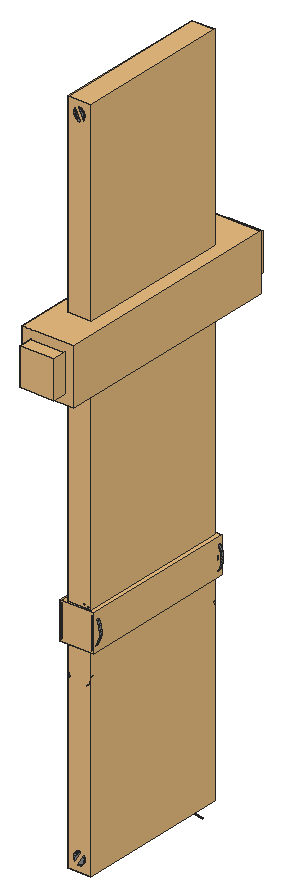
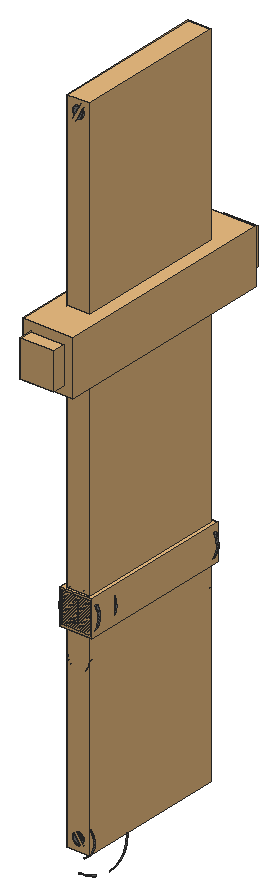
# SketchUp Ruby script. Lengths in inches.
U = 1.inch
M = Sketchup.active_model
def pt(a) = Geom::Point3d.new(a.map { |v| v * U })
def face(e, loops, mat)
  f = e.add_face(loops[0].map { |a| pt(a) })
  loops[1..].each { |l| e.add_face(l.map { |a| pt(a) }).erase! }
  f.material = f.back_material = mat if mat
  f
end
# faces: each face lists its corners as indices into pts; further lists are holes
def faces(e, pts, list, mat = nil) = list.each { |f| face(e, (f[0].is_a?(Array) ? f : [f]).map { |l| l.map { |i| pts[i] } }, mat) }
# xy, xz, yz: faces in a plane at the given z, y or x. An outline is a flat list of corners, or four numbers for a rectangle; further outlines are holes
def ring(l) = l.size == 4 ? [[l[0], l[1]], [l[2], l[1]], [l[2], l[3]], [l[0], l[3]]] : l.each_slice(2).to_a
def flat(e, list, mat, &to3) = list.each { |f| face(e, (f[0].is_a?(Array) ? f : [f]).map { |l| ring(l).map { |u, v| to3.(u, v) } }, mat) }
def xy(e, z, list, mat = nil) = flat(e, list, mat) { |x, y| [x, y, z] }
def xz(e, y, list, mat = nil) = flat(e, list, mat) { |x, z| [x, y, z] }
def yz(e, x, list, mat = nil) = flat(e, list, mat) { |y, z| [x, y, z] }
def lines(e, pts, list) = list.each { |a, b| e.add_line(pt(pts[a]), pt(pts[b])) }
# prism: a flat outline (further loops are holes) pulled along v
def prism(e, loops, v, mat = nil)
  f = face(e, loops, mat); d = Geom::Vector3d.new(v.map { |x| x * U })
  f.pushpull(f.normal.samedirection?(d) ? d.length : -d.length)
end
def box(e, o, s, mat = nil) = prism(e, [[o, [o[0] + s[0], o[1], o[2]], [o[0] + s[0], o[1] + s[1], o[2]], [o[0], o[1] + s[1], o[2]]]], [0, 0, s[2]], mat)
def at(x, y, z, deg = 0) = Geom::Transformation.translation(pt([x, y, z])) * Geom::Transformation.rotation(ORIGIN, Z_AXIS, deg.degrees)
def axes(o, x, y, z) = Geom::Transformation.new([*x, 0, *y, 0, *z, 0, *pt(o).to_a, 1])
def part(name) = M.definitions.add(name)
# library, detail: a bought-in or finely detailed component or shape, given as its bounding box
def library(name, o, s) = part(name).tap { |d| box(d.entities, o, s) }
def detail(e, o, s) = box(e.add_group.entities, o, s)
def put(e, d, t, mat = nil) = e.add_instance(d, t).tap { |i| i.material = mat if mat }
def group(e, t, mat = nil) = e.add_group.tap { |g| g.transformation = t; g.material = mat if mat }.entities
root = M.entities
M.materials.add("Material \#1").color = [140, 140, 140]
c1 = library("3DGeom~4_Defintion",[-18.02,-499.97,-221.16],[36.04,1000,262.12])
c2 = part("3DGeom~5_Defintion")
xy(c2.entities,-225.24,[[-0.79,-499.98,-2.33,-499.64,7.45,-496.14],[-0.79,-499.98,7.45,-496.14,1.58,-499.88],[1.58,-499.88,7.45,-496.14,3.84,-499.16],[-2.33,-499.64,7.4,-485.75,7.45,-496.14],[3.84,-499.16,7.45,-496.14,5.85,-497.89],
  [7.45,-496.14,7.4,-485.75,8.24,-487.08],[7.45,-496.14,8.24,-487.08,8.96,-489.34],[7.45,-496.14,8.96,-489.34,9.0625,-491.71],[7.45,-496.14,9.0625,-491.71,8.55,-494.03],[-7.4,-496.08,-8.24,-494.76,2.32,-482.2],
  [-8.24,-494.76,-8.96,-492.5,2.32,-482.2],[-8.96,-492.5,-9.0625,-490.125,2.32,-482.2],[-9.0625,-490.125,-8.55,-487.81,2.32,-482.2],[-8.55,-487.81,-7.45,-485.7,2.32,-482.2],[-7.45,-485.7,-5.85,-483.95,2.32,-482.2],
  [-5.85,-483.95,-3.84,-482.68,2.32,-482.2],[-3.84,-482.68,-1.58,-481.96,2.32,-482.2],[2.32,-482.2,-1.58,-481.96,0.79,-481.86],[0,481.82,-2.35,482.13,-6.92,496.71],[0,481.82,-6.92,496.71,1.55,482.04],
  [-2.35,482.13,-4.55,483.04,-6.92,496.71],[-4.55,483.04,-6.43,484.49,-6.92,496.71],[-6.43,484.49,-7.88,486.37,-6.92,496.71],[6.92,485.12,-1.55,499.8125,7.88,495.47],[6.92,485.12,7.88,495.47,7.88,486.37],
  [-7.88,486.37,-8.79,488.57,-6.92,496.71],[7.88,486.37,7.88,495.47,8.79,488.57],[-8.79,488.57,-9.1,490.92,-6.92,496.71],[8.79,488.57,7.88,495.47,9.1,490.92],[-9.1,490.92,-8.79,493.28,-6.92,496.71],
  [9.1,490.92,7.88,495.47,8.79,493.28],[-8.79,493.28,-7.88,495.47,-6.92,496.71],[7.88,495.47,-1.55,499.8125,0,500.02],[7.88,495.47,0,500.02,2.35,499.71],[7.88,495.47,2.35,499.71,4.55,498.8],
  [7.88,495.47,4.55,498.8,6.43,497.35]],"Material \#1")
xy(c2.entities,-221.57,[[-2.33,-499.64,-5.22,-498.37,7.4,-485.75],[-5.22,-498.37,-7.4,-496.08,5.22,-483.47],[-5.22,-498.37,5.22,-483.47,7.4,-485.75],[-7.4,-496.08,2.32,-482.2,5.22,-483.47],[1.55,482.04,-6.92,496.71,-4.55,498.8],
  [1.55,482.04,-4.55,498.8,4.55,483.04],[4.55,483.04,-4.55,498.8,-1.55,499.8125],[4.55,483.04,-1.55,499.8125,6.92,485.12]],"Material \#1")
xy(c2.entities,38.05,[[-2.33,-499.64,7.4,-485.75,-5.22,-498.37],[-5.22,-498.37,5.22,-483.47,-7.4,-496.08],[-5.22,-498.37,7.4,-485.75,5.22,-483.47],[-7.4,-496.08,5.22,-483.47,2.32,-482.2],[1.55,482.04,-4.55,498.8,-6.92,496.71],
  [1.55,482.04,4.55,483.04,-4.55,498.8],[4.55,483.04,-1.55,499.8125,-4.55,498.8],[4.55,483.04,6.92,485.12,-1.55,499.8125]],"Material \#1")
xy(c2.entities,41.72,[[-0.79,-499.98,7.45,-496.14,-2.33,-499.64],[-0.79,-499.98,1.58,-499.88,7.45,-496.14],[1.58,-499.88,3.84,-499.16,7.45,-496.14],[-2.33,-499.64,7.45,-496.14,7.4,-485.75],[3.84,-499.16,5.85,-497.89,7.45,-496.14],
  [7.45,-496.14,8.24,-487.08,7.4,-485.75],[7.45,-496.14,8.55,-494.03,9.0625,-491.71],[7.45,-496.14,8.96,-489.34,8.24,-487.08],[7.45,-496.14,9.0625,-491.71,8.96,-489.34],[-7.4,-496.08,2.32,-482.2,-8.24,-494.76],
  [-8.24,-494.76,2.32,-482.2,-8.96,-492.5],[-8.96,-492.5,2.32,-482.2,-9.0625,-490.125],[-9.0625,-490.125,2.32,-482.2,-8.55,-487.81],[-8.55,-487.81,2.32,-482.2,-7.45,-485.7],[-7.45,-485.7,2.32,-482.2,-5.85,-483.95],
  [-5.85,-483.95,2.32,-482.2,-3.84,-482.68],[-3.84,-482.68,2.32,-482.2,-1.58,-481.96],[2.32,-482.2,0.79,-481.86,-1.58,-481.96],[0,481.82,-6.92,496.71,-2.35,482.13],[0,481.82,1.55,482.04,-6.92,496.71],
  [-2.35,482.13,-6.92,496.71,-4.55,483.04],[-4.55,483.04,-6.92,496.71,-6.43,484.49],[-6.43,484.49,-6.92,496.71,-7.88,486.37],[6.92,485.12,7.88,495.47,-1.55,499.8125],[6.92,485.12,7.88,486.37,7.88,495.47],
  [-7.88,486.37,-6.92,496.71,-8.79,488.57],[7.88,486.37,8.79,488.57,7.88,495.47],[-8.79,488.57,-6.92,496.71,-9.1,490.92],[8.79,488.57,9.1,490.92,7.88,495.47],[-9.1,490.92,-6.92,496.71,-8.79,493.28],
  [9.1,490.92,8.79,493.28,7.88,495.47],[-8.79,493.28,-6.92,496.71,-7.88,495.47],[7.88,495.47,0,500.02,-1.55,499.8125],[7.88,495.47,2.35,499.71,0,500.02],[7.88,495.47,4.55,498.8,2.35,499.71],
  [7.88,495.47,6.43,497.35,4.55,498.8]],"Material \#1")
c3 = library("3DGeom~12_Defintion",[-95.68,-755.75,-830.03],[191.36,191.37,1000])
c4 = part("3DGeom~10_Defintion")
yz(c4.entities,-68.96,[[-797.08,-844.83,-797.08,-827.59,-922.41,-827.59],[-922.41,-844.83,-797.08,-844.83,-922.41,-827.59]],"Material \#1")
yz(c4.entities,68.97,[[-922.41,-844.83,-797.08,-827.59,-797.08,-844.83],[-922.41,-844.83,-922.41,-827.59,-797.08,-827.59],[-797.08,137.93,-922.41,155.17,-797.08,155.17],[-922.41,137.93,-922.41,155.17,-797.08,137.93]],"Material \#1")
p = [[-15.8,-989.55,-844.83],[-15.8,-989.55,-827.59],[0,-991.38,-827.59],[0,-991.38,-844.83],[15.8,-989.55,-827.59],[15.8,-989.55,-844.83],
  [-30.32,-984.36,-844.83],[-30.32,-984.36,-827.59],[30.31,-984.36,-827.59],[30.31,-984.36,-844.83],[-43.12,-976.21,-844.83],[-43.12,-976.21,-827.59],
  [43.12,-976.21,-827.59],[43.12,-976.21,-844.83],[-53.81,-965.53,-844.83],[-53.81,-965.53,-827.59],[53.8,-965.53,-827.59],[53.8,-965.53,-844.83],
  [-61.95,-952.73,-844.83],[-61.95,-952.73,-827.59],[53.8,-965.53,-827.59],[61.95,-952.73,-827.59],[61.95,-952.73,-844.83],[-67.15,-938.21,-844.83],
  [-67.15,-938.21,-827.59],[67.14,-938.21,-827.59],[67.14,-938.21,-844.83],[-68.96,-922.41,-844.83],[-68.96,-922.41,-827.59],[67.14,-938.21,-827.59],
  [68.97,-922.41,-827.59],[68.97,-922.41,-844.83],[-69.1,-794.86,-844.83],[-69.1,-794.86,-827.59],[-68.96,-797.08,-827.59],[-68.96,-797.08,-844.83],
  [68.97,-797.08,-844.83],[68.97,-797.08,-827.59],[69.11,-794.71,-827.59],[69.11,-794.71,-844.83],[-69.48,-792.73,-844.83],[-69.48,-792.73,-827.59],
  [69.53,-792.51,-827.59],[69.53,-792.51,-844.83],[-70.14,-790.6875,-844.83],[-70.14,-790.6875,-827.59],[70.24,-790.48,-827.59],[70.24,-790.48,-844.83],
  [-71.08,-788.73,-844.83],[-71.08,-788.73,-827.59],[71.22,-788.57,-827.59],[71.22,-788.57,-844.83],[-72.32,-786.86,-844.83],[-72.32,-786.86,-827.59],
  [72.47,-786.78,-827.59],[72.47,-786.78,-844.83],[-73.8,-785.17,-844.83],[-73.8,-785.17,-827.59],[74,-785.04,-827.59],[74,-785.04,-844.83],
  [-75.96,-783.21,-844.83],[-75.96,-783.21,-827.59],[74,-785.04,-827.59],[75.76,-783.39,-827.59],[75.76,-783.39,-844.83],[86.625,-772.95,-827.59],
  [86.61,-772.96,-844.83],[-86.89,-773.25,-844.83],[-86.89,-773.25,-827.59],[-75.96,-783.21,-844.83],[-96.66,-761.8,-844.83],[-96.66,-761.8,-827.59],
  [86.625,-772.95,-827.59],[86.63,-772.94,-844.83],[86.61,-772.96,-844.83],[86.625,-772.95,-827.59],[86.62,-772.95,-827.59],[86.62,-772.95,-827.59],
  [96.31,-761.375,-827.59],[96.31,-761.375,-844.83],[86.63,-772.94,-844.83],[86.625,-772.95,-827.59],[86.62,-772.95,-827.59],[-104.96,-749.18,-844.83],
  [-104.96,-749.18,-827.59],[-96.66,-761.8,-827.59],[-96.66,-761.8,-844.83],[96.31,-761.375,-827.59],[104.62,-748.77,-827.59],[104.62,-748.77,-844.83],
  [-111.64,-735.52,-844.83],[-111.64,-735.52,-827.59],[111.39,-735.21,-827.59],[111.39,-735.21,-844.83],[-116.49,-721.23,-844.83],[-116.49,-721.23,-827.59],
  [116.4375,-720.78,-827.59],[116.4375,-720.78,-844.83],[-119.64,-705.62,-844.83],[-119.64,-705.62,-827.59],[119.6,-705.57,-827.59],[119.6,-705.57,-844.83],
  [-120.6875,-689.65,-844.83],[-120.6875,-689.65,-827.59],[120.69,-689.65,-827.59],[120.69,-689.65,-844.83],[-117.5,-662,-844.83],[-117.5,-662,-827.59],
  [117.5,-662,-827.59],[117.5,-662,-844.83],[-108.41,-636.61,-844.83],[-108.41,-636.61,-827.59],[117.5,-662,-844.83],[108.41,-636.61,-827.59],
  [108.41,-636.61,-844.83],[-93.91,-613.95,-844.83],[-93.91,-613.95,-827.59],[-108.41,-636.61,-827.59],[108.41,-636.61,-844.83],[94.16,-614.19,-827.59],
  [94.16,-614.19,-844.83],[94.16,-614.19,-827.59],[75.46,-595.5,-827.59],[75.46,-595.5,-844.83],[-75.46,-595.5,-844.83],[-75.46,-595.5,-827.59],
  [-93.91,-613.95,-827.59],[-93.91,-613.95,-827.59],[-93.91,-613.95,-844.83],[-53.05,-581.24,-844.83],[-53.05,-581.24,-827.59],[-75.46,-595.5,-827.59],
  [-75.46,-595.5,-844.83],[53.05,-581.24,-827.59],[53.05,-581.24,-844.83],[-27.65,-572.16,-844.83],[-27.65,-572.16,-827.59],[-53.05,-581.24,-827.59],
  [-53.05,-581.24,-844.83],[27.66,-572.16,-827.59],[27.66,-572.16,-844.83],[0,-568.97,-844.83],[0,-568.97,-827.59],[-27.65,-572.16,-827.59],
  [-27.65,-572.16,-844.83],[0,-568.97,-844.83],[-15.8,-989.55,155.17],[0,-991.38,155.17],[0,-991.38,137.93],[-15.8,-989.55,137.93],
  [15.8,-989.55,155.17],[15.8,-989.55,137.93],[-30.32,-984.36,155.17],[-30.32,-984.36,137.93],[30.31,-984.36,155.17],[30.31,-984.36,137.93],
  [-43.125,-976.22,155.17],[-43.125,-976.22,137.93],[43.12,-976.22,155.17],[43.12,-976.22,137.93],[-53.81,-965.53,155.17],[-53.81,-965.53,137.93],
  [53.8,-965.53,155.17],[53.8,-965.53,137.93],[-61.96,-952.73,155.17],[-61.95,-952.73,137.93],[61.95,-952.73,155.17],[61.95,-952.73,137.93],
  [53.8,-965.53,137.93],[-67.15,-938.21,155.17],[-67.15,-938.21,137.93],[67.14,-938.21,155.17],[67.14,-938.21,137.93],[-68.96,-922.41,155.17],
  [-68.96,-922.41,137.93],[68.97,-922.41,155.17],[68.97,-922.41,137.93],[67.14,-938.21,137.93],[-68.97,-797.08,155.17],[-68.97,-797.08,137.93],
  [-69.1,-794.86,155.17],[-69.1,-794.86,137.93],[68.97,-797.08,155.17],[69.11,-794.71,155.17],[69.11,-794.71,137.93],[68.97,-797.08,137.93],
  [-69.48,-792.73,155.17],[-69.48,-792.73,137.93],[69.53,-792.51,155.17],[69.53,-792.51,137.93],[-70.14,-790.6875,155.17],[-70.14,-790.6875,137.93],
  [70.24,-790.48,155.17],[70.24,-790.48,137.93],[-71.08,-788.73,155.17],[-71.08,-788.73,137.93],[71.22,-788.57,155.17],[71.22,-788.57,137.93],
  [-72.32,-786.86,155.17],[-72.32,-786.86,137.93],[72.47,-786.78,155.17],[72.47,-786.78,137.93],[-73.8,-785.17,155.17],[-73.8,-785.17,137.93],
  [74,-785.04,155.17],[74,-785.04,137.93],[-75.96,-783.21,155.17],[-75.96,-783.21,137.93],[75.76,-783.39,155.17],[75.76,-783.39,137.93],
  [74,-785.04,137.93],[86.61,-772.96,155.17],[86.625,-772.95,137.93],[-86.88,-773.25,155.17],[-75.96,-783.21,155.17],[-86.88,-773.25,137.93],
  [-96.66,-761.8,155.17],[-96.66,-761.8,137.93],[86.63,-772.94,155.17],[86.625,-772.95,137.93],[86.61,-772.96,155.17],[86.62,-772.95,137.93],
  [86.625,-772.95,137.93],[96.31,-761.375,155.17],[96.31,-761.375,137.93],[86.62,-772.95,137.93],[86.63,-772.94,155.17],[86.62,-772.95,137.93],
  [86.625,-772.95,137.93],[-104.96,-749.18,155.17],[-96.66,-761.8,155.17],[-96.66,-761.8,137.93],[-104.96,-749.18,137.93],[104.62,-748.77,155.17],
  [104.62,-748.77,137.93],[96.31,-761.375,137.93],[-111.64,-735.52,155.17],[-111.64,-735.52,137.93],[111.39,-735.21,155.17],[111.39,-735.21,137.93],
  [-116.49,-721.23,155.17],[-116.49,-721.23,137.93],[116.4375,-720.78,155.17],[116.4375,-720.78,137.93],[-119.64,-705.62,155.17],[-119.64,-705.62,137.93],
  [119.6,-705.57,155.17],[119.6,-705.57,137.93],[-120.6875,-689.65,155.17],[-120.6875,-689.65,137.93],[120.69,-689.65,155.17],[120.69,-689.65,137.93],
  [-117.5,-662,155.17],[-117.5,-662,137.93],[117.5,-662,155.17],[117.5,-662,137.93],[-108.41,-636.61,155.17],[-108.41,-636.61,137.93],
  [117.5,-662,155.17],[108.41,-636.61,155.17],[108.41,-636.61,137.93],[-93.91,-613.95,155.17],[-108.41,-636.61,137.93],[-93.91,-613.95,137.93],
  [108.41,-636.61,155.17],[94.16,-614.19,155.17],[94.16,-614.19,137.93],[75.46,-595.5,155.17],[75.46,-595.5,137.93],[94.16,-614.19,137.93],
  [-75.46,-595.5,155.17],[-93.91,-613.95,155.17],[-93.91,-613.95,137.93],[-75.46,-595.5,137.93],[-53.05,-581.24,155.17],[-75.46,-595.5,155.17],
  [-75.46,-595.5,137.93],[-53.05,-581.24,137.93],[53.05,-581.24,155.17],[53.05,-581.24,137.93],[-27.65,-572.16,155.17],[-53.05,-581.24,155.17],
  [-53.05,-581.24,137.93],[-27.65,-572.16,137.93],[27.65,-572.16,155.17],[27.65,-572.16,137.93],[0,-568.97,155.17],[-27.65,-572.16,155.17],
  [-27.65,-572.16,137.93],[0,-568.97,137.93],[0,-568.97,155.17]]
faces(c4.entities,p,[[0,1,2],[2,3,0],[3,2,4],[4,5,3],[6,7,1],[1,0,6],[5,4,8],[8,9,5],
  [10,11,7],[7,6,10],[9,8,12],[12,13,9],[14,15,11],[11,10,14],[13,12,16],[16,17,13],
  [18,19,15],[15,14,18],[17,20,21],[21,22,17],[23,24,19],[19,18,23],[22,21,25],[25,26,22],
  [27,28,24],[24,23,27],[26,29,30],[30,31,26],[32,33,34],[34,35,32],[36,37,38],[38,39,36],
  [40,41,33],[33,32,40],[39,38,42],[42,43,39],[44,45,41],[41,40,44],[43,42,46],[46,47,43],
  [48,49,45],[45,44,48],[47,46,50],[50,51,47],[52,53,49],[49,48,52],[51,50,54],[54,55,51],
  [56,57,53],[53,52,56],[55,54,58],[58,59,55],[60,61,57],[57,56,60],[59,62,63],[63,64,59],
  [64,63,65],[65,66,64],[67,68,61],[61,69,67],[70,71,68],[68,67,70],[72,73,66],[74,75,76],
  [73,77,78],[78,79,73],[80,81,82],[83,84,85],[85,86,83],[79,87,88],[88,89,79],[90,91,84],
  [84,83,90],[89,88,92],[92,93,89],[94,95,91],[91,90,94],[93,92,96],[96,97,93],[98,99,95],
  [95,94,98],[97,96,100],[100,101,97],[102,103,99],[99,98,102],[101,100,104],[104,105,101],[106,107,103],
  [103,102,106],[105,104,108],[108,109,105],[110,111,107],[107,106,110],[112,108,113],[113,114,112],[115,116,117],
  [117,110,115],[118,113,119],[119,120,118],[120,121,122],[122,123,120],[124,125,126],[127,128,124],[129,130,131],
  [131,132,129],[123,122,133],[133,134,123],[135,136,137],[137,138,135],[134,133,139],[139,140,134],[141,142,143],
  [143,144,141],[140,139,142],[142,145,140],[146,147,148],[148,149,146],[147,150,151],[151,148,147],[152,146,149],
  [149,153,152],[150,154,155],[155,151,150],[156,152,153],[153,157,156],[154,158,159],[159,155,154],[160,156,157],
  [157,161,160],[158,162,163],[163,159,158],[164,160,161],[161,165,164],[162,166,167],[167,168,162],[169,164,165],
  [165,170,169],[166,171,172],[172,167,166],[173,169,170],[170,174,173],[171,175,176],[176,177,171],[178,173,174],
  [174,179,178],[180,178,179],[179,181,180],[182,183,184],[184,185,182],[186,180,181],[181,187,186],[183,188,189],
  [189,184,183],[190,186,187],[187,191,190],[188,192,193],[193,189,188],[194,190,191],[191,195,194],[192,196,197],
  [197,193,192],[198,194,195],[195,199,198],[196,200,201],[201,197,196],[202,198,199],[199,203,202],[200,204,205],
  [205,201,200],[206,202,203],[203,207,206],[204,208,209],[209,210,204],[208,211,212],[212,209,208],[213,214,207],
  [207,215,213],[216,213,215],[215,217,216],[211,218,219],[220,221,222],[218,223,224],[224,225,218],[226,227,228],
  [229,230,231],[231,232,229],[223,233,234],[234,235,223],[236,229,232],[232,237,236],[233,238,239],[239,234,233],
  [240,236,237],[237,241,240],[238,242,243],[243,239,238],[244,240,241],[241,245,244],[242,246,247],[247,243,242],
  [248,244,245],[245,249,248],[246,250,251],[251,247,246],[252,248,249],[249,253,252],[250,254,255],[255,251,250],
  [256,252,253],[253,257,256],[258,259,260],[260,255,258],[261,256,262],[262,263,261],[264,265,266],[266,260,264],
  [265,267,268],[268,269,265],[270,271,272],[272,273,270],[274,275,276],[276,277,274],[267,278,279],[279,268,267],
  [280,281,282],[282,283,280],[278,284,285],[285,279,278],[286,287,288],[288,289,286],[284,290,289],[289,285,284]],"Material \#1")
c5 = library("3DGeom~14_Defintion",[-102.17,352.37,-727.27],[204.35,204.35,1000])
c6 = library("3DGeom~13_Defintion",[-84.91,-744.98,-830.03],[169.82,169.83,1000])
c7 = library("3DGeom~1_Defintion",[-60.87,347.29,-704.08],[121.74,121.75,1000])
xy(root,40.525,[[109.178,198.412,109.209,198.412,109.178,198.724],[109.209,198.412,109.209,198.724,109.178,198.724]],"Material \#1")
xy(root,40.839,[[109.162,198.412,109.162,198.724,109.214,198.724],[109.162,198.412,109.214,198.724,109.214,198.412]],"Material \#1")
xz(root,197.036,[[109.138,40.912,109.188,40.949,109.188,40.918]],"Material \#1")
xz(root,198.379,[[109.188,40.003,109.128,40.018,109.157,40.007],[109.188,40.003,109.248,40.018,109.128,40.018],[109.128,40.018,109.051,40.438,109.054,40.118],[109.128,40.018,109.322,40.118,109.051,40.438],[109.128,40.018,109.054,40.118,109.081,40.059],
  [109.128,40.018,109.081,40.059,109.102,40.036],[109.081,40.059,109.054,40.118,109.065,40.087],[109.322,40.118,109.046,40.46,109.048,40.455],[109.322,40.118,109.048,40.455,109.05,40.45],[109.322,40.118,109.05,40.45,109.051,40.444],
  [109.054,40.118,109.051,40.438,109.051,40.152],[109.322,40.118,109.051,40.444,109.051,40.438],[109.325,40.152,109.019,40.535,109.046,40.46],[109.325,40.152,109.053,40.498,109.019,40.535],[109.325,40.152,109.093,40.471,109.053,40.498],
  [109.325,40.152,109.138,40.453,109.093,40.471],[109.046,40.46,108.945,40.647,109.042,40.466],[109.046,40.46,108.993,40.579,108.945,40.647],[109.046,40.46,109.019,40.535,108.993,40.579],[109.042,40.466,108.945,40.647,109.039,40.47],
  [109.039,40.47,108.945,40.647,108.991,40.523],[109.039,40.47,108.991,40.523,109.034,40.475],[109.034,40.475,108.991,40.523,109.011,40.497],[108.991,40.523,108.945,40.647,108.961,40.581],[108.991,40.523,108.961,40.581,108.975,40.551],
  [108.993,40.579,108.977,40.628,108.945,40.647],[108.961,40.581,108.945,40.647,108.951,40.613],[108.977,40.628,108.971,40.682,108.945,40.647],[108.945,40.647,108.949,40.743,108.943,40.682],[108.945,40.647,108.971,40.682,108.977,40.736],
  [108.945,40.647,108.977,40.736,108.993,40.786],[108.945,40.647,108.993,40.786,108.996,40.849],[108.945,40.647,108.996,40.849,108.949,40.743],[108.949,40.743,108.996,40.849,108.967,40.8],[108.993,40.786,109.019,40.829,108.996,40.849],
  [109.019,40.829,109.053,40.866,108.996,40.849],[108.996,40.849,109.053,40.866,109.093,40.894],[108.996,40.849,109.08,40.922,109.035,40.89],[108.996,40.849,109.093,40.894,109.188,40.949],[108.996,40.849,109.188,40.949,109.08,40.922],
  [109.093,40.894,109.138,40.912,109.188,40.949],[109.138,40.912,109.188,40.918,109.188,40.949],[109.08,40.922,109.188,40.949,109.132,40.942]],"Material \#1")
xz(root,198.412,[[109.178,40.525,109.167,40.549,109.199,40.549],[109.178,40.525,109.199,40.549,109.209,40.525],[109.167,40.549,109.162,40.557,109.204,40.557],[109.167,40.549,109.204,40.557,109.199,40.549],[109.162,40.557,109.162,40.574,109.204,40.574],
  [109.162,40.557,109.204,40.574,109.204,40.557],[109.162,40.574,109.167,40.582,109.199,40.582],[109.162,40.574,109.199,40.582,109.204,40.574],[109.167,40.582,109.167,40.612,109.209,40.612],[109.167,40.582,109.209,40.612,109.199,40.582],
  [109.167,40.612,109.167,40.639,109.209,40.639],[109.167,40.612,109.209,40.639,109.209,40.612],[109.167,40.639,109.159,40.661,109.217,40.661],[109.167,40.639,109.217,40.661,109.209,40.639],[109.159,40.661,109.159,40.684,109.217,40.684],
  [109.159,40.661,109.217,40.684,109.217,40.661],[109.159,40.684,109.167,40.706,109.209,40.706],[109.159,40.684,109.209,40.706,109.217,40.684],[109.167,40.706,109.162,40.721,109.214,40.721],[109.167,40.706,109.214,40.721,109.209,40.706],
  [109.162,40.721,109.162,40.773,109.214,40.773],[109.162,40.721,109.214,40.773,109.214,40.721],[109.162,40.773,109.169,40.776,109.208,40.776],[109.162,40.773,109.208,40.776,109.214,40.773],[109.169,40.776,109.169,40.784,109.208,40.784],
  [109.169,40.776,109.208,40.784,109.208,40.776],[109.169,40.784,109.162,40.788,109.214,40.788],[109.169,40.784,109.214,40.788,109.208,40.784],[109.162,40.788,109.162,40.839,109.214,40.839],[109.162,40.788,109.214,40.839,109.214,40.788]],"Material \#1")
xz(root,198.647,[[109.188,40.447,109.132,40.455,109.188,40.455],[109.188,40.447,109.188,40.455,109.242,40.462],[109.188,40.447,109.242,40.462,109.244,40.455],[109.132,40.455,109.08,40.478,109.134,40.462],[109.132,40.455,109.134,40.462,109.188,40.455],
  [109.244,40.455,109.242,40.462,109.293,40.485],[109.244,40.455,109.293,40.485,109.296,40.478],[109.134,40.462,109.08,40.478,109.083,40.485],[109.08,40.478,109.035,40.516,109.083,40.485],[109.296,40.478,109.293,40.485,109.336,40.521],
  [109.296,40.478,109.336,40.521,109.341,40.516],[109.083,40.485,109.035,40.516,109.04,40.521],[109.035,40.516,109,40.564,109.04,40.521],[109.341,40.516,109.336,40.521,109.369,40.568],[109.341,40.516,109.369,40.568,109.376,40.564],
  [109.04,40.521,109,40.564,109.007,40.568],[109,40.564,108.979,40.621,109.007,40.568],[109.376,40.564,109.369,40.568,109.39,40.623],[109.376,40.564,109.39,40.623,109.397,40.621],[109.007,40.568,108.979,40.621,108.986,40.623],
  [108.979,40.621,108.971,40.682,108.986,40.623],[109.397,40.621,109.39,40.623,109.397,40.682],[109.397,40.621,109.397,40.682,109.405,40.682],[108.986,40.623,108.971,40.682,108.979,40.682],[108.971,40.682,108.979,40.743,108.979,40.682],
  [108.979,40.682,108.979,40.743,108.986,40.741],[109.397,40.682,109.39,40.741,109.405,40.682],[109.405,40.682,109.39,40.741,109.397,40.743],[108.986,40.741,108.979,40.743,109,40.8],[108.986,40.741,109,40.8,109.007,40.796],
  [109.39,40.741,109.369,40.796,109.397,40.743],[109.397,40.743,109.369,40.796,109.376,40.8],[109.007,40.796,109,40.8,109.035,40.849],[109.007,40.796,109.035,40.849,109.04,40.843],[109.369,40.796,109.336,40.843,109.376,40.8],
  [109.376,40.8,109.336,40.843,109.341,40.849],[109.04,40.843,109.035,40.849,109.08,40.886],[109.04,40.843,109.08,40.886,109.083,40.879],[109.336,40.843,109.293,40.879,109.341,40.849],[109.341,40.849,109.293,40.879,109.296,40.886],
  [109.083,40.879,109.08,40.886,109.132,40.91],[109.083,40.879,109.132,40.91,109.134,40.902],[109.293,40.879,109.242,40.902,109.296,40.886],[109.296,40.886,109.242,40.902,109.244,40.91],[109.134,40.902,109.132,40.91,109.188,40.918],
  [109.134,40.902,109.188,40.918,109.188,40.91],[109.242,40.902,109.188,40.91,109.244,40.91],[109.188,40.91,109.188,40.918,109.244,40.91]],"Material \#1")
xz(root,198.681,[[109.188,37.641,109.074,37.652,109.188,37.652],[109.074,37.652,108.968,37.684,109.076,37.663],[109.074,37.652,109.076,37.663,109.188,37.652],[109.076,37.663,108.968,37.684,108.972,37.695],[108.781,37.802,108.705,37.885,108.788,37.811],
  [108.788,37.811,108.705,37.885,108.713,37.893],[109.115,37.839,109.082,37.855,109.119,37.85],[109.119,37.85,109.082,37.855,109.088,37.866],[109.082,37.855,109.053,37.878,109.088,37.866],[109.088,37.866,109.053,37.878,109.06,37.887],
  [109.053,37.878,109.028,37.905,109.06,37.887],[108.705,37.885,108.646,37.975,108.713,37.893],[109.06,37.887,109.028,37.905,109.036,37.913],[108.713,37.893,108.646,37.975,108.655,37.981],[109.028,37.905,109.007,37.937,109.036,37.913],
  [109.036,37.913,109.007,37.937,109.016,37.943],[109.007,37.937,108.991,37.973,109.016,37.943],[109.016,37.943,108.991,37.973,109.002,37.977],[108.991,37.973,108.982,38.011,109.002,37.977],[108.646,37.975,108.596,38.088,108.655,37.981],
  [109.002,37.977,108.982,38.011,108.992,38.014],[108.655,37.981,108.596,38.088,108.606,38.092],[108.982,38.011,108.978,38.048,108.992,38.014],[108.992,38.014,108.978,38.048,108.989,38.048],[108.978,38.048,108.982,38.093,108.989,38.048],
  [108.989,38.048,108.982,38.093,108.992,38.091],[108.596,38.088,108.567,38.204,108.606,38.092],[108.992,38.091,108.982,38.093,108.991,38.132],[108.992,38.091,108.991,38.132,109.002,38.128],[108.606,38.092,108.567,38.204,108.577,38.206],
  [109.002,38.128,108.991,38.132,109.007,38.167],[109.002,38.128,109.007,38.167,109.016,38.161],[109.016,38.161,109.007,38.167,109.028,38.199],[109.016,38.161,109.028,38.199,109.036,38.192],[109.036,38.192,109.028,38.199,109.053,38.227],
  [109.036,38.192,109.053,38.227,109.06,38.218],[108.567,38.204,108.556,38.331,108.577,38.206],[108.577,38.206,108.556,38.331,108.567,38.332],[109.06,38.218,109.053,38.227,109.082,38.249],[109.06,38.218,109.082,38.249,109.088,38.239],
  [109.088,38.239,109.082,38.249,109.115,38.266],[109.088,38.239,109.115,38.266,109.119,38.255],[109.119,38.255,109.115,38.266,109.151,38.277],[109.119,38.255,109.151,38.277,109.152,38.265],[109.152,38.265,109.151,38.277,109.188,38.28]],"Material \#1")
yz(root,109.162,[[198.412,40.788,198.724,40.839,198.412,40.839]],"Material \#1")
yz(root,109.167,[[198.412,40.582,198.724,40.612,198.412,40.612]],"Material \#1")
p = [[109.1,198.674,37.962],[109.1,198.647,37.962],[109.118,198.647,37.944],[109.118,198.674,37.944],[109.14,198.647,37.931],[109.14,198.674,37.931],
  [109.156,198.654,37.956],[109.156,198.681,37.956],[109.116,198.681,37.986],[109.116,198.654,37.986],[109.206,198.684,38.127],[109.206,198.657,38.127],
  [109.13,198.657,38.008],[109.13,198.684,38.008],[109.17,198.657,37.978],[109.17,198.684,37.978],[109.246,198.657,38.097],[109.246,198.684,38.097],
  [109.236,198.674,38.173],[109.236,198.647,38.174],[109.22,198.654,38.149],[109.261,198.681,38.118],[109.261,198.654,38.118],[109.276,198.647,38.143],
  [109.276,198.674,38.143],[109.258,198.647,38.161],[109.258,198.674,38.161],[109.22,198.681,38.149],[109.165,198.724,40.553],[109.162,198.412,40.557],
  [109.167,198.412,40.549],[109.165,198.724,40.553],[109.167,198.412,40.549],[109.178,198.412,40.525],[109.178,198.724,40.525],[109.165,198.724,40.553],
  [109.202,198.724,40.553],[109.199,198.412,40.549],[109.204,198.412,40.557],[109.159,198.724,40.672],[109.159,198.412,40.661],[109.167,198.412,40.639],
  [109.165,198.724,40.578],[109.162,198.412,40.574],[109.162,198.412,40.557],[109.165,198.724,40.553],[109.167,198.412,40.639],[109.163,198.724,40.65],
  [109.159,198.724,40.672],[109.165,198.724,40.578],[109.167,198.412,40.582],[109.162,198.412,40.574],[109.163,198.724,40.65],[109.167,198.412,40.639],
  [109.167,198.412,40.612],[109.167,198.412,40.612],[109.167,198.724,40.612],[109.163,198.724,40.65],[109.167,198.412,40.582],[109.165,198.724,40.578],
  [109.167,198.724,40.612],[109.202,198.724,40.578],[109.204,198.412,40.574],[109.199,198.412,40.582],[109.202,198.724,40.553],[109.204,198.412,40.557],
  [109.204,198.412,40.574],[109.202,198.724,40.578],[109.202,198.724,40.578],[109.199,198.412,40.582],[109.209,198.412,40.612],[109.163,198.724,40.695],
  [109.159,198.412,40.684],[109.159,198.412,40.661],[109.159,198.412,40.661],[109.159,198.724,40.672],[109.163,198.724,40.695],[109.159,198.412,40.684],
  [109.163,198.724,40.695],[109.165,198.724,40.714],[109.165,198.724,40.777],[109.162,198.412,40.773],[109.162,198.412,40.721],[109.162,198.412,40.721],
  [109.162,198.724,40.725],[109.165,198.724,40.777],[109.165,198.724,40.714],[109.167,198.412,40.706],[109.159,198.412,40.684],[109.162,198.724,40.725],
  [109.162,198.412,40.721],[109.167,198.412,40.706],[109.167,198.412,40.706],[109.165,198.724,40.714],[109.162,198.724,40.725],[109.162,198.412,40.788],
  [109.165,198.724,40.777],[109.162,198.724,40.839],[109.212,198.724,40.782],[109.214,198.412,40.773],[109.208,198.412,40.776],[109.165,198.724,40.777],
  [109.169,198.412,40.784],[109.169,198.412,40.776],[109.165,198.724,40.777],[109.162,198.412,40.788],[109.165,198.724,40.777],[109.162,198.412,40.773],
  [109.212,198.724,40.782],[109.208,198.412,40.784],[109.214,198.412,40.788],[109.212,198.724,40.782],[109.213,198.681,46.353],[109.213,198.654,46.353],
  [109.226,198.647,46.327],[109.226,198.674,46.327],[109.249,198.647,46.337],[109.249,198.674,46.337],[109.269,198.647,46.354],[109.269,198.674,46.354],
  [109.255,198.654,46.38],[109.134,198.684,46.502],[109.134,198.657,46.502],[109.2,198.657,46.376],[109.2,198.684,46.376],[109.255,198.681,46.38],
  [109.243,198.657,46.403],[109.243,198.684,46.403],[109.176,198.657,46.528],[109.176,198.684,46.528],[109.107,198.674,46.551],[109.107,198.647,46.551],
  [109.121,198.654,46.525],[109.121,198.681,46.525],[109.164,198.654,46.552],[109.164,198.681,46.552],[109.15,198.647,46.578],[109.15,198.674,46.578],
  [109.127,198.647,46.567],[109.127,198.674,46.567]]
faces(root,p,[[0,1,2],[2,3,0],[3,2,4],[4,5,3],[5,4,6],[6,7,5],[8,9,1],[1,0,8],
  [10,11,12],[12,13,10],[13,12,9],[9,8,13],[7,6,14],[14,15,7],[15,14,16],[16,17,15],
  [18,19,20],[21,22,23],[23,24,21],[24,23,25],[25,26,24],[17,16,22],[22,21,17],[20,27,18],
  [27,20,11],[11,10,27],[26,25,19],[19,18,26],[28,29,30],[31,32,33],[33,34,35],[36,37,38],
  [39,40,41],[42,43,44],[44,45,42],[46,47,48],[49,50,51],[52,53,54],[55,56,57],[58,59,60],
  [61,62,63],[64,65,66],[66,67,64],[68,69,70],[71,72,73],[74,75,76],[77,78,79],[80,81,82],
  [83,84,85],[86,87,88],[89,90,91],[92,93,94],[95,96,97],[98,99,100],[101,102,103],[104,105,102],
  [106,103,107],[108,109,110],[111,100,109],[112,113,114],[114,115,112],[115,114,116],[116,117,115],[117,116,118],
  [118,119,117],[119,118,120],[121,122,123],[123,124,121],[124,123,113],[113,112,124],[125,120,126],[126,127,125],
  [127,126,128],[128,129,127],[120,125,119],[130,131,132],[132,133,130],[133,132,122],[122,121,133],[129,128,134],
  [134,135,129],[135,134,136],[136,137,135],[137,136,138],[138,139,137],[139,138,131],[131,130,139]],"Material \#1")
put(root,c1,axes([109.1875,197.04,42.25],[0.00802,0,0],[0,0,0.00871],[0,-0.00745,0]),"Material \#1")
put(root,c2,axes([109.1875,197.04,42.25],[0.00787,0,0],[0,0,0.00856],[0,-0.00732,0]),"Material \#1")
put(root,c3,axes([109.1875,197.04,42.25],[0.00219,0,0],[0,0,0.00238],[0,-0.00203,0]),"Material \#1")
put(root,c4,axes([109.1875,197.04,42.25],[0.00209,0,0],[0,0,0.00228],[0,-0.00195,0]),"Material \#1")
put(root,c5,axes([109.1875,197.04,42.25],[0.00318,0,0],[0,0,0.00345],[0,-0.00295,0]),"Material \#1")
put(root,c6,axes([109.1875,197.04,42.25],[0.00219,0,0],[0,0,0.00238],[0,-0.00203,0]),"Material \#1")
put(root,c7,axes([109.1875,197.04,42.25],[0.00354,0,0],[0,0,0.00385],[0,-0.00329,0]),"Material \#1")
